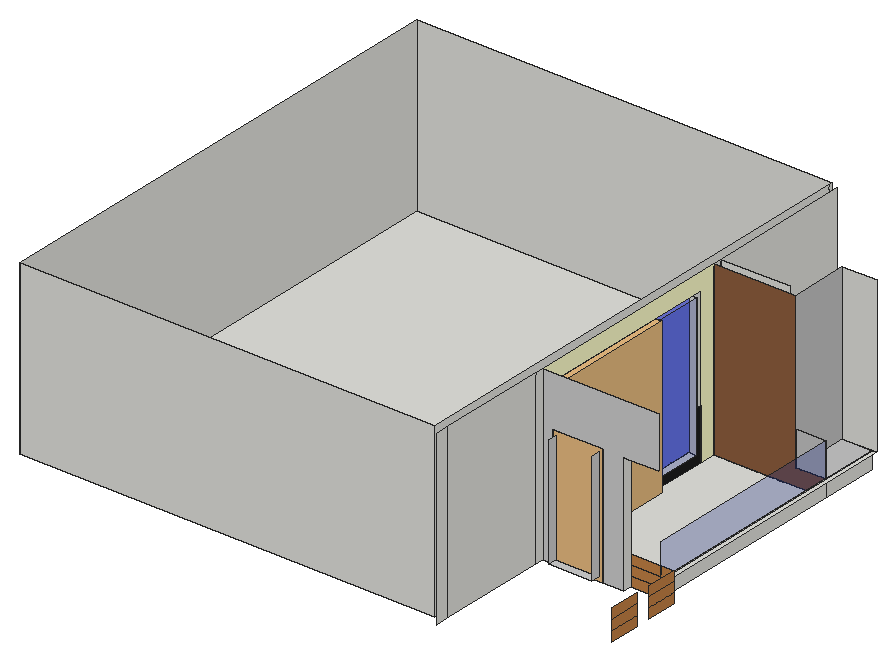
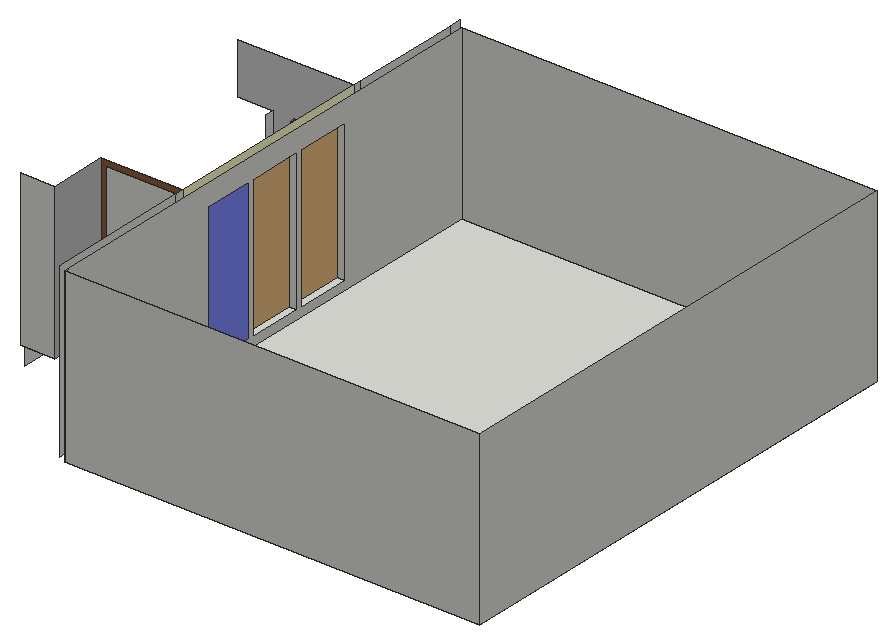
# SketchUp Ruby script. Lengths in inches.
U = 1.inch
M = Sketchup.active_model
def pt(a) = Geom::Point3d.new(a.map { |v| v * U })
def face(e, loops, mat)
  f = e.add_face(loops[0].map { |a| pt(a) })
  loops[1..].each { |l| e.add_face(l.map { |a| pt(a) }).erase! }
  f.material = f.back_material = mat if mat
  f
end
# faces: each face lists its corners as indices into pts; further lists are holes
def faces(e, pts, list, mat = nil) = list.each { |f| face(e, (f[0].is_a?(Array) ? f : [f]).map { |l| l.map { |i| pts[i] } }, mat) }
# xy, xz, yz: faces in a plane at the given z, y or x. An outline is a flat list of corners, or four numbers for a rectangle; further outlines are holes
def ring(l) = l.size == 4 ? [[l[0], l[1]], [l[2], l[1]], [l[2], l[3]], [l[0], l[3]]] : l.each_slice(2).to_a
def flat(e, list, mat, &to3) = list.each { |f| face(e, (f[0].is_a?(Array) ? f : [f]).map { |l| ring(l).map { |u, v| to3.(u, v) } }, mat) }
def xy(e, z, list, mat = nil) = flat(e, list, mat) { |x, y| [x, y, z] }
def xz(e, y, list, mat = nil) = flat(e, list, mat) { |x, z| [x, y, z] }
def yz(e, x, list, mat = nil) = flat(e, list, mat) { |y, z| [x, y, z] }
def lines(e, pts, list) = list.each { |a, b| e.add_line(pt(pts[a]), pt(pts[b])) }
# prism: a flat outline (further loops are holes) pulled along v
def prism(e, loops, v, mat = nil)
  f = face(e, loops, mat); d = Geom::Vector3d.new(v.map { |x| x * U })
  f.pushpull(f.normal.samedirection?(d) ? d.length : -d.length)
end
def box(e, o, s, mat = nil) = prism(e, [[o, [o[0] + s[0], o[1], o[2]], [o[0] + s[0], o[1] + s[1], o[2]], [o[0], o[1] + s[1], o[2]]]], [0, 0, s[2]], mat)
def at(x, y, z, deg = 0) = Geom::Transformation.translation(pt([x, y, z])) * Geom::Transformation.rotation(ORIGIN, Z_AXIS, deg.degrees)
def axes(o, x, y, z) = Geom::Transformation.new([*x, 0, *y, 0, *z, 0, *pt(o).to_a, 1])
def part(name) = M.definitions.add(name)
# library, detail: a bought-in or finely detailed component or shape, given as its bounding box
def library(name, o, s) = part(name).tap { |d| box(d.entities, o, s) }
def detail(e, o, s) = box(e.add_group.entities, o, s)
def put(e, d, t, mat = nil) = e.add_instance(d, t).tap { |i| i.material = mat if mat }
def group(e, t, mat = nil) = e.add_group.tap { |g| g.transformation = t; g.material = mat if mat }.entities
root = M.entities
M.materials.add("E01_Mint_Frost").color = [255, 255, 204]
M.materials.add("Embossed_Stainless_Steel_2_1K").color = [196, 196, 196]
M.materials.add("Glass_Basic_01").color = [23, 48, 186]
M.materials["Glass_Basic_01"].alpha = 0.25
M.materials.add("I03_Bluebell_Mist").color = [130, 140, 255]
M.materials.add("LightPink_Translucent").color = [144, 107, 117]
M.materials["LightPink_Translucent"].alpha = 0.75
M.materials.add("M08_Obsidian_Black").color = [30, 30, 30]
M.materials.add("Wood_Floor_01_1K").color = [196, 130, 70]
M.materials.add("Wood_Veneer_15_1K").color = [142, 95, 62]
M.materials.add("[Cladding_Siding_White]1").color = [207, 207, 207]
c1 = library("porta+4",[0.2,-5.42,1.33],[46.55,4.72,83.21])
c2 = library("mesh-166",[-1553.69,-2604.3125,-42.18],[1702.88,1401.6,88.28])
c3 = part("blade")
p = [[2.15,0.21,22],[0,0.17,0],[0.09,0.45,0],[2.18,0.31,22],[2.29,0.31,22],[0.38,0.45,0],
  [2.48,0.24,33],[2.49,0.24,33],[2.48,0.22,33]]
faces(c3.entities,p,[[0,1,2,3],[4,5,2,3],[6,3,4,7],[8,0,3,6]])
c4 = part("seeds")
p = [[0.3,-0.1,1.38],[-0.01,-0.03,1.59],[-0.01,-0.03,0.03],[0.14,-0.07,-0.07],[0.29,-0.03,3],[0.15,0.01,3.11]]
faces(c4.entities,p,[[0,1,2,3],[1,0,4,5]],"LightPink_Translucent")
c5 = part("blade with seeds")
put(c5.entities,c3,at(0,0,0))
put(c5.entities,c4,axes([2.4,0.25,30.99],[1.5799,-0.05474,1.17369],[-0.12525,1.92788,0.29478],[-0.07173,-0.02425,1.56792]))
xy(root,276,[[6,6,297,354],[303,93,360,93,360,99,381,99,381,243,303,243],[303,243,351,249]])
xy(root,279,[[312,87,342,93]],"[Cladding_Siding_White]1")
xy(root,282,[[297,108,303,147],[297,150,303,189],[297,192,303,228]])
xy(root,288,[[381,99,384,283.95]])
xy(root,288,[[360,243,381,283.95]],"Embossed_Stainless_Steel_2_1K")
xz(root,6,[[6,276,297,396]])
xz(root,93,[[303,276,303,396,384,396,384,360,360,360,360,276,345,276,345,360,309,360,309,276],[[309,276,345,360],[312,279,342,357]]],"[Cladding_Siding_White]1")
xz(root,99,[[381,276,384,283],[381,283,384,288]])
xz(root,99,[[360,276,381,283],[384,276,390,283],[360,283,381,290],[384,283,384,288,381,288,381,290,390,290,390,283],[360,290,381,297],
  [381,290,390,297]],"Wood_Floor_01_1K")
xz(root,108,[[297,282,303,381]])
xz(root,147,[[297,282,303,381]])
xz(root,150,[[297,282,303,381]])
xz(root,189,[[297,282,303,381]])
xz(root,192,[[297,282,303,381]])
xz(root,228,[[297,282,303,381]])
xz(root,243,[[360,288,381,312]],"Embossed_Stainless_Steel_2_1K")
xz(root,243,[[303,276,381,276,381,288,360,288,360,396,303,396]],"Wood_Veneer_15_1K")
xz(root,249,[[303,276,351,396]])
xz(root,283.95,[[360,288,384,396]])
xz(root,354,[[6,276,297,396]])
yz(root,6,[[6,276,354,396]])
yz(root,297,[[[6,276,351,396],[108,282,147,381],[150,282,189,381],[192,282,228,381]],[351,276,354,396]])
yz(root,297,[[192,282,228,381]],"I03_Bluebell_Mist")
yz(root,303,[[0,276,9,396],[9,276,87,396],[87,276,93,396],[243,276,249,396],[249,276,351,396]])
yz(root,303,[[93,276,192,276,192,312,189,312,189,282,150,282,150,312,147,312,147,282,108,282,108,312,105,312,105,384,231,384,231,276,243,276,243,396,93,396]],"E01_Mint_Frost")
yz(root,303,[[192,282,228,381]],"Glass_Basic_01")
yz(root,303,[[192,276,231,276,231,312,228,312,228,282,192,282]],"M08_Obsidian_Black")
yz(root,312,[[87,279,93,357]],"[Cladding_Siding_White]1")
yz(root,342,[[87,279,93,357]],"[Cladding_Siding_White]1")
yz(root,360,[[93,276,99,360]])
yz(root,360,[[243,288,283.95,396]],"Embossed_Stainless_Steel_2_1K")
yz(root,381,[[99,276,243,288],[243,276,283.95,288]])
yz(root,381,[[99,288,243,312]],"Glass_Basic_01")
yz(root,390,[[45,276,66.6,283],[77.4,276,99,283],[45,283,66.6,290],[77.4,283,99,290],[45,290,66.6,297],
  [77.4,290,99,297]],"Wood_Floor_01_1K")
p = [[303,231,312],[303,231,276]]
lines(root,p,[[0,1]])
put(root,c1,axes([310,97.01,274.61],[0.74,0,0],[0,0.74,0],[0,0,1.01007]))
g1 = group(root,at(305.35,127.3,410.45))
put(g1,c2,axes([-0.18,-15.08,66.23],[0,-0.05118,0],[0,0,0.07706],[-0.05118,0,0]))
put(root,c5,axes([329.04,108.57,288.76],[-0.2011,-0.61905,-0.65645],[0.5793,-0.22295,-0.17229],[-0.02223,-0.20963,1.449]))
put(root,c5,axes([330.88,109.625,288.76],[0.17956,0.55272,-0.65059],[-0.51723,0.19906,-0.17075],[0.01985,0.18717,1.43607]))
put(root,c5,axes([330.82,108.47,288.73],[0.50939,0.09897,-0.58612],[-0.10749,0.61051,-0.15383],[0.15202,0.07398,1.29375]))
put(root,c5,axes([329.12,109.73,288.73],[-0.50939,-0.09897,-0.58612],[0.10749,-0.61051,-0.15383],[-0.15202,-0.07398,1.29375]))
put(root,c5,axes([329.92,107.9375,288.73],[0.32983,-0.45375,-0.58612],[0.40974,0.41145,-0.15383],[0.13217,-0.11319,1.29375]))
put(root,c5,axes([330.02,110.26,288.73],[-0.32983,0.45375,-0.58612],[-0.40974,-0.41145,-0.15383],[-0.13217,0.11319,1.29375]))
put(root,c5,axes([331.49,107.3125,288.6875],[0.4583,0.30184,-0.46672],[-0.27394,0.54125,0],[0.10438,0.06875,1.48054]))
put(root,c5,axes([330.57,111.5,288.6875],[-0.4583,0.30184,-0.46672],[-0.27394,-0.54125,0],[-0.10438,0.06875,1.48054]))
put(root,c5,axes([327.85,108.49,288.6875],[0,-0.60368,-0.46672],[0.54787,0,0],[0,-0.13749,1.48054]))
put(root,c5,axes([328.45,110.89,288.6875],[-0.4583,-0.30184,-0.46672],[0.27394,-0.54125,0],[-0.10438,-0.06875,1.48054]))
put(root,c5,axes([329.375,106.7,288.6875],[0.4583,-0.30184,-0.46672],[0.27394,0.54125,0],[0.10438,-0.06875,1.48054]))
put(root,c5,axes([332.09,109.71,288.6875],[0,0.60368,-0.46672],[-0.54787,0,0],[0,0.13749,1.48054]))
put(root,c5,axes([329.34,108.73,288.87],[0.23759,-0.54397,-0.42055],[0.49367,0.26179,0.2024],[0,-0.12539,1.35025]))
put(root,c5,axes([329.38,109.54,288.87],[-0.29417,-0.5067,-0.42055],[0.44558,-0.35681,0.2024],[-0.0952,-0.0627,1.35025]))
put(root,c5,axes([330.5625,108.66,288.87],[0.29417,0.5067,-0.42055],[-0.44558,0.35681,0.2024],[0.0952,0.0627,1.35025]))
put(root,c5,axes([330.6,109.46,288.87],[-0.23759,0.54397,-0.42055],[-0.49367,-0.26179,0.2024],[0,0.12539,1.35025]))
put(root,c5,axes([330.01,109.9,288.87],[-0.53176,0.03727,-0.42055],[-0.04809,-0.6186,0.2024],[-0.0952,0.0627,1.35025]))
put(root,c5,axes([329.48,106.9375,288.7],[0.45686,0.14937,-0.29119],[-0.11503,0.52602,0.29119],[0.0921,-0.06066,1.30635]))
put(root,c5,axes([331.85,109.69,288.7],[-0.34183,0.37665,-0.29119],[-0.34183,-0.37665,0.29119],[0,0.12132,1.30635]))
put(root,c5,axes([328.58,110.66,288.7],[-0.11503,-0.52602,-0.29119],[0.45686,-0.14937,0.29119],[-0.0921,-0.06066,1.30635]))
put(root,c5,axes([330.46,111.26,288.7],[-0.45686,-0.14937,-0.29119],[0.11503,-0.52602,0.29119],[-0.0921,0.06066,1.30635]))
put(root,c5,axes([331.37,107.54,288.7],[0.11503,0.52602,-0.29119],[-0.45686,0.14937,0.29119],[0.0921,0.06066,1.30635]))
put(root,c5,axes([328.09,108.5,288.7],[0.34183,-0.37665,-0.29119],[0.34183,0.37665,0.29119],[0,-0.12132,1.30635]))
put(root,c5,axes([331.47,111.61,288.2],[0.03568,-0.08715,1.65762],[0.44916,-0.25668,-0.25323],[0.13617,0.13285,0.28235]))
put(root,c5,axes([327.48,108.87,288.2],[0.01242,0.09514,1.65762],[-0.25036,0.49684,-0.25323],[-0.17783,-0.02504,0.28235]))
put(root,c5,axes([329.72,105.64,288.2],[-0.08214,0.02175,1.65762],[-0.45422,-0.24483,-0.25323],[0.00762,-0.20421,0.28235]))
put(root,c5,axes([329.37,111.59,288.2],[0.07925,-0.03285,1.65762],[0.47671,0.18081,-0.25323],[0.01394,0.20378,0.28235]))
put(root,c5,axes([332.76,108.96,288.2],[-0.02559,-0.09165,1.65762],[0.1775,-0.53611,-0.25323],[0.17905,-0.00771,0.28235]))
put(root,c5,axes([328.25,106.39,288.2],[-0.04743,0.07953,1.65762],[-0.47936,0.17146,-0.25323],[-0.1158,-0.15598,0.28235]))
put(root,c5,axes([327.35,111.53,288.2],[0.06569,0.06031,1.65762],[0.11138,0.55882,-0.25323],[-0.14558,0.11917,0.28235]))
put(root,c5,axes([331.73,106.68,288.2],[-0.07329,-0.04756,1.65762],[-0.18827,-0.53132,-0.25323],[0.127,-0.14418,0.28235]))
put(root,c5,axes([329,108.02,288.29],[-0.482,0.24169,1.21193],[-0.15342,-0.69348,0.47091],[0.29598,0.01154,1.37843]))
put(root,c5,axes([330.38,109.73,289.3],[0.05706,0.68884,-0.2735],[-0.59432,0.04165,-0.47002],[-0.10465,0.09176,1.50125]))
put(root,c5,axes([330.66,109.01,289.3],[0.55148,0.28805,-0.2735],[-0.26554,0.60796,-0.47002],[0.01733,0.14927,1.50125]))
put(root,c5,axes([329.29,109.1875,289.3],[-0.55148,-0.28805,-0.2735],[0.26554,-0.60796,-0.47002],[-0.01733,-0.14927,1.50125]))
put(root,c5,axes([329.5625,108.46,289.3],[-0.05706,-0.68884,-0.2735],[0.59432,-0.04165,-0.47002],[0.10465,-0.09176,1.50125]))
put(root,c5,axes([330.25,108.375,289.3],[0.49442,-0.40079,-0.2735],[0.32878,0.56631,-0.47002],[0.12199,0.05751,1.50125]))
put(root,c5,axes([329.69,109.82,289.3],[-0.49442,0.40079,-0.2735],[-0.32878,-0.56631,-0.47002],[-0.12199,-0.05751,1.50125]))
put(root,c5,axes([330.55,110.42,288.85],[0.51411,-0.20483,-0.18046],[0.18065,0.59003,0.00007],[0.05675,-0.02264,1.63463]))
put(root,c5,axes([330.25,110,289.11],[-0.47817,-0.48589,-0.23681],[0.40236,-0.54561,0.51822],[-0.12876,0.05684,1.58123]))
put(root,c5,axes([329.42,109.83,289.08],[0.12979,-0.71533,-0.22023],[0.6154,0.12469,0.48194],[-0.10753,-0.09879,1.47054]))
put(root,c5,axes([329.63,106.07,288.79],[-0.3384,0.34633,-0.03659],[-0.31006,-0.3793,-0.1659],[-0.02183,-0.10747,0.54722]))
put(root,c5,axes([327.95,106.7,288.79],[-0.14126,0.49294,-0.03659],[-0.43477,-0.15163,-0.1659],[-0.06601,-0.08063,0.54722]))
put(root,c5,axes([332.99,108.83,288.92],[-0.3036,-0.38602,-0.06098],[0.3325,-0.3537,-0.27651],[0.09421,-0.0249,0.91203]))
put(root,c5,axes([332.42,109.34,288.65],[-0.3154,0.07245,1.33088],[-0.0502,-0.57666,0.07618],[0.2209,-0.08728,0.75732]))
put(root,c5,axes([330.6,111.33,288.85],[-0.30235,-0.60704,-0.04834],[0.51222,-0.33735,0.48511],[-0.12622,0.0578,1.53813]))
put(root,c5,axes([331.98,109.6,288.86],[-0.61202,-0.00483,-0.04678],[0,-0.67471,0.46946],[-0.01923,0.15359,1.48851]))
put(root,c5,axes([330.22,110.51,288.95],[0.2129,0.69353,-0.05652],[-0.60833,0.24302,0],[0.00743,0.02422,1.61843]))
put(root,c5,axes([330.36,109.42,288.95],[-0.45549,-0.5196,-0.05763],[0.45577,-0.51991,0],[-0.01591,-0.01814,1.65037]))
put(root,c5,axes([330.52,109.16,288.95],[0,0.69816,-0.05299],[-0.61233,0,0],[0,0.02194,1.68606]))
put(root,c5,axes([328.96,106.79,289.02],[-0.30616,-0.60492,0],[0.51222,-0.33735,-0.48511],[0.11666,-0.07683,1.53889]))
put(root,c5,axes([328.73,111.25,289.02],[-0.30616,0.60492,0],[-0.51222,-0.33735,-0.48511],[-0.11666,-0.07683,1.53889]))
put(root,c5,axes([330.98,111.4,289.02],[0.30616,0.60492,0],[-0.51222,0.33735,-0.48511],[-0.11666,0.07683,1.53889]))
put(root,c5,axes([327.72,108.95,289.02],[-0.61233,0,0],[0,-0.67471,-0.48511],[0,-0.15367,1.53889]))
put(root,c5,axes([331.21,106.95,289.03],[0.30616,-0.60492,0],[0.51222,0.33735,-0.48511],[0.11666,0.07683,1.53889]))
put(root,c5,axes([332.23,109.25,289.03],[0.61233,0,0],[0,0.67471,-0.48511],[0,0.15367,1.53889]))
put(root,c5,axes([328.19,108.77,288.98],[-0.45549,0.50754,0.28911],[-0.45577,-0.5022,-0.34302],[-0.01591,-0.14413,1.54992]))
put(root,c5,axes([330.61,111.02,288.98],[0.61306,0.19622,0.28911],[-0.15337,0.70136,-0.34302],[-0.10147,0.08778,1.54992]))
put(root,c5,axes([329.84,110.72,288.86],[-0.49367,-0.27103,0],[0.23759,-0.56315,0],[0,0,1.52945]))
put(root,c5,axes([330.4,110.73,288.86],[0.49367,0.27103,0],[-0.23759,0.56315,0],[0,0,1.64456]))
put(root,c5,axes([329.95,110.49,288.86],[-0.15978,-0.52046,0],[0.45625,-0.18226,0],[0,0,1.45109]))
put(root,c5,axes([330.21,108.875,288.86],[0,-0.69851,0],[0.61233,0,0],[0,0,1.68689]))
put(root,c5,axes([330.625,109.03,288.87],[0.54787,0,0],[0,0.62498,0],[0,0,1.67702]))
put(root,c5,axes([330.61,109.3,288.875],[0.34183,0.38994,0],[-0.34183,0.38994,0],[0,0,1.5911]))
put(root,c5,axes([329.5,109.48,289.01],[0.61893,0.12719,0.43009],[-0.12596,0.71835,0.16877],[-0.09045,-0.06936,1.49325]))
put(root,c5,axes([329.92,108.4375,289.01],[-0.40602,0.54785,0.43009],[-0.48237,-0.48361,0.16877],[0.09788,-0.05467,1.49325]))
put(root,c5,axes([329.44,108.82,289.01],[0.2129,0.67504,0.43009],[-0.60833,0.23474,0.16877],[0.00743,-0.12404,1.49325]))
put(root,c5,axes([330.45,108.71,289.03],[-0.61893,-0.12719,0.46247],[0.12596,-0.71835,0.18148],[0.09045,0.06936,1.60565]))
put(root,c5,axes([329.64,109,289.08],[0.55175,0.29259,0.22621],[-0.26554,0.60796,0.47002],[0,-0.14015,1.5091]))
put(root,c5,axes([330.49,109.87,289.25],[0.36178,0.36271,0.13611],[-0.30177,0.40921,-0.38866],[-0.084,0.05532,1.1914]))
put(root,c5,axes([330.29,108.2,289.25],[0.09447,-0.53876,0.13611],[0.46155,0.09352,-0.38866],[0.084,0.05532,1.1914]))
put(root,c5,axes([330.8125,108.97,289.25],[0.45625,-0.17605,0.13611],[0.15978,0.50273,-0.38866],[0,0.11064,1.1914]))
put(root,c5,axes([329.65,109.99,289.25],[-0.09447,0.53876,0.13611],[-0.46155,-0.09352,-0.38866],[-0.084,-0.05532,1.1914]))
put(root,c5,axes([328.28,111.67,289.45],[0.44486,-0.1069,0.06117],[0.10227,0.43069,-0.81126],[-0.0282,0.21802,0.72719]))
put(root,c5,axes([327.82,107.74,289.23],[0.09561,0.16807,1.34422],[-0.22031,0.45686,-0.28909],[-0.22622,-0.1092,0.57472]))
put(root,c5,axes([328.17,112.125,289.23],[0.15453,-0.09523,1.34422],[0.38153,0.28715,-0.28909],[-0.11356,0.24846,0.57472]))
put(root,c5,axes([330.41,110.78,289.23],[0.00864,-0.20012,1.34422],[0.41296,-0.22353,-0.28909],[0.12748,0.23952,0.57472]))
put(root,c5,axes([330.75,106.31,289.23],[-0.13919,0.12219,1.34422],[-0.41687,-0.21387,-0.28909],[0.07727,-0.26598,0.57472]))
put(root,c5,axes([332.1,107.74,289.23],[-0.17494,-0.01788,1.34422],[-0.17922,-0.47967,-0.28909],[0.21491,-0.13569,0.57472]))
put(root,c5,axes([328.6,106.07,289.23],[-0.02965,0.19748,1.34422],[-0.43351,0.16532,-0.28909],[-0.10133,-0.25525,0.57472]))
put(root,c5,axes([332.51,110.19,289.23],[-0.11793,-0.14847,1.34422],[0.15345,-0.49116,-0.28909],[0.23861,0.06653,0.57472]))
put(root,c5,axes([327.16,110.19,289.23],[0.17018,0.04956,1.34422],[0.10969,0.50618,-0.28909],[-0.23117,0.09475,0.57472]))
put(root,c5,axes([330.78,107.57,289.12],[-0.52621,0.16023,0.16584],[-0.12993,-0.59629,0.32981],[0.04693,0.08688,1.50782]))
put(root,c5,axes([331.54,109.13,289.12],[-0.38474,-0.43973,0.16584],[0.38772,-0.42651,0.32981],[-0.04249,0.0898,1.50782]))
put(root,c5,axes([329.21,107.53,289.12],[-0.14146,0.59996,0.16584],[-0.51766,-0.16978,0.32981],[0.08942,-0.00292,1.50782]))
put(root,c5,axes([330.73,110.66,289.12],[0.14146,-0.59996,0.16584],[0.51766,0.16978,0.32981],[-0.08942,0.00292,1.50782]))
put(root,c5,axes([329.16,110.63,289.12],[0.52621,-0.16023,0.16584],[0.12993,0.59629,0.32981],[-0.04693,-0.08688,1.50782]))
put(root,c5,axes([328.09,109.05,289.12],[0,0.60368,0.46672],[-0.54787,0,0],[0,-0.13749,1.48054]))
put(root,c5,axes([330.95,107.26,289.12],[-0.4583,-0.30184,0.46672],[0.27394,-0.54125,0],[0.10438,0.06875,1.48054]))
put(root,c5,axes([331.85,109.15,289.12],[0,-0.60368,0.46672],[0.54787,0,0],[0,0.13749,1.48054]))
put(root,c5,axes([330.875,110.98,289.12],[0.4583,-0.30184,0.46672],[0.27394,0.54125,0],[-0.10438,0.06875,1.48054]))
put(root,c5,axes([328.99,110.93,289.12],[0.4583,0.30184,0.46672],[-0.27394,0.54125,0],[-0.10438,-0.06875,1.48054]))
put(root,c5,axes([330.61,108.84,289.35],[0.23759,-0.54397,0.42055],[0.49367,0.26179,-0.2024],[0,0.12539,1.35025]))
put(root,c5,axes([329.46,108.6,289.35],[-0.53176,0.03727,0.42055],[-0.04809,-0.6186,-0.2024],[0.0952,-0.0627,1.35025]))
put(root,c5,axes([330.1,108.34,289.35],[-0.29417,-0.5067,0.42055],[0.44558,-0.35681,-0.2024],[0.0952,0.0627,1.35025]))
put(root,c5,axes([329.34,109.35,289.35],[-0.23759,0.54397,0.42055],[-0.49367,-0.26179,-0.2024],[0,-0.12539,1.35025]))
put(root,c5,axes([330.48,109.6,289.35],[0.53176,-0.03727,0.42055],[0.04809,0.6186,-0.2024],[-0.0952,0.0627,1.35025]))
put(root,c5,axes([331.4375,111.75,289.3],[-0.31402,-0.01893,0.98757],[0.20738,-0.40212,0.54525],[0.12405,0.14286,0.77466]))
put(root,c5,axes([327.25,108.24,289.39],[0.31263,-0.0432,1.07969],[-0.19831,0.38061,0.79328],[-0.15449,-0.0571,0.23781]))
put(root,c5,axes([331.39,110.96,289.39],[-0.27572,-0.17358,1.07969],[0.35602,-0.17637,0.79328],[0.09603,0.1494,0.23781]))
put(root,c5,axes([326.81,111.25,289.39],[0.20408,-0.2736,1.07969],[0.08053,0.43313,0.79328],[-0.14748,0.07756,0.23781]))
put(root,c5,axes([333.08,109.53,289.39],[-0.30256,0.09966,1.07969],[0.14242,-0.41189,0.79328],[0.16051,0.02818,0.23781]))
put(root,c5,axes([328.45,105.76,289.39],[0.25544,0.21011,1.07969],[-0.37201,0.1263,0.79328],[-0.0796,-0.16148,0.23781]))
put(root,c5,axes([328.54,112.44,289.39],[-0.01267,-0.35895,1.07969],[0.31667,0.25602,0.79328],[-0.06228,0.17109,0.23781]))
put(root,c5,axes([332.3,106.86,289.39],[-0.16311,0.3073,1.07969],[-0.1402,-0.41288,0.79328],[0.13471,-0.10346,0.23781]))
put(root,c5,axes([330.24,105.33,289.39],[0.06282,0.35202,1.07969],[-0.34848,-0.19497,0.79328],[0.0375,-0.18025,0.23781]))
put(root,c5,axes([330.72,109.01,289.46],[-0.01338,-0.56839,1.32796],[0.60542,0.14734,0.56227],[-0.14319,0.31102,1.25349]))
put(root,c5,axes([329.07,106.87,291.47],[-0.41756,-0.29179,-0.66783],[0.29675,-0.51132,0.08059],[-0.15128,-0.17422,0.9447]))
put(root,c5,axes([329.52,111.35,291.47],[0.23372,0.49086,-0.66783],[-0.48111,0.27356,0.08059],[0.05465,0.23717,0.9447]))
put(root,c5,axes([328.22,107.59,291.47],[-0.48951,-0.01454,-0.66783],[0.03288,-0.61207,0.08059],[-0.20738,-0.06459,0.9447]))
put(root,c5,axes([331.72,108.18,291.47],[0.25579,-0.47633,-0.66783],[0.44823,0.33852,0.08059],[0.15273,-0.17258,0.9447]))
put(root,c5,axes([331.85,109.38,291.47],[0.4303,-0.26662,-0.66783],[0.23981,0.54882,0.08059],[0.20791,-0.06234,0.9447]))
put(root,c5,axes([331.09,107.21,291.47],[0.01274,-0.55841,-0.66783],[0.53656,0.0375,0.08059],[0.05662,-0.23657,0.9447]))
put(root,c5,axes([331.43,110.49,291.47],[0.48951,0.01454,-0.66783],[-0.03288,0.61207,0.08059],[0.20738,0.06459,0.9447]))
put(root,c5,axes([330.12,106.73,291.47],[-0.23372,-0.49086,-0.66783],[0.48111,-0.27356,0.08059],[-0.05465,-0.23717,0.9447]))
put(root,c5,axes([329.7,111.45,291.19],[0.48137,0.15133,-0.48033],[-0.165,0.51886,-0.37205],[0.04414,0.2089,0.91906]))
put(root,c5,axes([330.98,107.02,291.19],[-0.35055,-0.40562,-0.48033],[0.37031,-0.35523,-0.37205],[0.05334,-0.20609,0.91906]))
put(root,c5,axes([328.87,106.88,291.19],[-0.48321,0.1435,-0.48033],[-0.08453,-0.54345,-0.37205],[-0.12979,-0.15574,0.91906]))
put(root,c5,axes([331.93,109.18,291.19],[0.13266,-0.54912,-0.48033],[0.45484,0.18822,-0.37205],[0.18313,-0.05035,0.91906]))
put(root,c5,axes([328.05,107.71,291.19],[-0.35558,0.39989,-0.48033],[-0.31141,-0.42243,-0.37205],[-0.18066,-0.06084,0.91906]))
put(root,c5,axes([327.93,110.125,291.19],[0.1258,0.55122,-0.48033],[-0.4764,0.09643,-0.37205],[-0.13652,0.14806,0.91906]))
put(root,c5,axes([327.71,108.9,291.19],[-0.13266,0.54912,-0.48033],[-0.45484,-0.18822,-0.37205],[-0.18313,0.05035,0.91906]))
put(root,c5,axes([329.94,106.63,291.19],[-0.48137,-0.15133,-0.48033],[0.165,-0.51886,-0.37205],[-0.04414,-0.2089,0.91906]))
put(root,c5,axes([331.71,107.96,291.19],[-0.1258,-0.55122,-0.48033],[0.4764,-0.09643,-0.37205],[0.13652,-0.14806,0.91906]))
put(root,c5,axes([330.77,111.2,291.19],[0.48321,-0.1435,-0.48033],[0.08453,0.54345,-0.37205],[0.12979,0.15574,0.91906]))
put(root,c5,axes([328.55,110.875,291.81],[-0.01274,0.55841,-0.74129],[-0.53656,-0.0375,0.08946],[-0.05662,0.23657,1.04862]))
put(root,c5,axes([328.66,111.06,291.5],[0.35055,0.40562,-0.53317],[-0.37031,0.35523,-0.41298],[-0.05334,0.20609,1.02016]))
put(root,c5,axes([330.07,110.17,289.92],[0.42317,0.24343,1.42185],[-0.41456,0.52443,0.56227],[-0.18569,-0.31082,1.19198]))
put(root,c5,axes([328.67,108.57,289.93],[0.13919,-0.08733,1.6644],[0.048,0.60974,0.13026],[-0.3015,0.08091,0.59487]))
put(root,c5,axes([328.37,111.66,289.95],[0.01076,-0.31164,1.45085],[0.48391,0.16461,0.20049],[-0.04193,0.33214,0.68509]))
put(root,c5,axes([331.72,110.74,291.05],[0.27863,0.37797,-0.33289],[-0.31815,0.35779,0.42977],[0.16164,0.05444,0.82232]))
put(root,c5,axes([327.43,108.65,291.05],[-0.40696,-0.16841,-0.33289],[0.1187,-0.49132,0.42977],[-0.16385,0.04505,0.82232]))
put(root,c5,axes([327.58,110.07,291.05],[-0.42626,0.08628,-0.33289],[-0.11256,-0.4932,0.42977],[-0.12215,0.13247,0.82232]))
put(root,c5,axes([332.21,109.43,291.05],[0.40696,0.16841,-0.33289],[-0.1187,0.49132,0.42977],[0.16385,-0.04505,0.82232]))
put(root,c5,axes([328.92,106.48,291.05],[-0.07563,-0.48625,-0.33289],[0.43235,-0.1284,0.42977],[-0.11613,-0.13934,0.82232]))
put(root,c5,axes([328.33,111.21,291.05],[-0.33133,0.31784,-0.33289],[-0.31365,-0.36292,0.42977],[-0.04772,0.1844,0.82232]))
put(root,c5,axes([332.0625,108.02,291.05],[0.42626,-0.08628,-0.33289],[0.11256,0.4932,0.42977],[0.12215,-0.13247,0.82232]))
put(root,c5,axes([329.48,111.77,291.05],[-0.14763,0.46424,-0.33289],[-0.4307,-0.1354,0.42977],[0.03949,0.18691,0.82232]))
put(root,c5,axes([331.3125,106.875,291.05],[0.33133,-0.31784,-0.33289],[0.31365,0.36292,0.42977],[0.04772,-0.1844,0.82232]))
put(root,c5,axes([330.16,106.3125,291.05],[0.14763,-0.46424,-0.33289],[0.4307,0.1354,0.42977],[-0.03949,-0.18691,0.82232]))
put(root,c5,axes([327.92,107.34,291.05],[-0.27863,-0.37797,-0.33289],[0.31815,-0.35779,0.42977],[-0.16164,-0.05444,0.82232]))
put(root,c5,axes([332.55,110.8,290.49],[-0.09372,-0.50747,-0.03282],[0.44299,-0.11666,-0.14882],[0.09251,0.03217,0.49085]))
put(root,c5,axes([330.72,109.78,290.44],[-0.1819,-0.10401,1.61094],[0.37643,-0.43634,0.13026],[0.23461,0.19684,0.68866]))
put(root,c5,axes([330.49,106.93,290.44],[-0.09118,0.2075,1.61094],[-0.3825,-0.42941,0.13026],[0.17255,-0.26763,0.68866]))
put(root,c5,axes([331.1,108.82,290.44],[-0.20312,0.01367,1.61094],[0.13474,-0.59258,0.13026],[0.28946,0.03665,0.68866]))
put(root,c5,axes([329.97,110.38,290.44],[-0.11194,-0.19382,1.61094],[0.51725,-0.16318,0.13026],[0.1169,0.30428,0.68866]))
put(root,c5,axes([329.06,110.48,290.44],[-0.01199,-0.2317,1.61094],[0.51947,0.15371,0.13026],[-0.03213,0.3302,0.68866]))
put(root,c5,axes([328.22,110.04,290.44],[0.09118,-0.2075,1.61094],[0.3825,0.42941,0.13026],[-0.17255,0.26763,0.68866]))
put(root,c5,axes([327.69,109.18,290.44],[0.16991,-0.12769,1.61094],[0.14304,0.59005,0.13026],[-0.26674,0.13336,0.68866]))
put(root,c5,axes([328.3125,109.58,290.44],[0.12231,-0.18549,1.61094],[0.30882,0.50067,0.13026],[-0.21182,0.22801,0.68866]))
put(root,c5,axes([328.74,106.59,290.44],[0.11194,0.19382,1.61094],[-0.51725,0.16318,0.13026],[-0.1169,-0.30428,0.68866]))
put(root,c5,axes([327.99,107.19,290.44],[0.1819,0.10401,1.61094],[-0.37643,0.43634,0.13026],[-0.23461,-0.19684,0.68866]))
put(root,c5,axes([327.61,108.14,290.44],[0.20312,-0.01367,1.61094],[-0.13474,0.59258,0.13026],[-0.28946,-0.03665,0.68866]))
put(root,c5,axes([331.4,110.79,291.52],[0.02622,-0.61393,-0.11431],[0.49645,0.01678,-0.63445],[0.1912,0.04265,0.96403]))
put(root,c5,axes([327.6875,108.43,291.52],[0.24639,0.54664,-0.11431],[-0.43729,0.26863,-0.63445],[-0.18428,0.07212,0.96403]))
put(root,c5,axes([331.35,107.24,291.52],[-0.53819,-0.02991,-0.11431],[0.01471,-0.56632,-0.63445],[0.03738,-0.21811,0.96403]))
put(root,c5,axes([331.96,109.65,291.52],[-0.24639,-0.54664,-0.11431],[0.43729,-0.26863,-0.63445],[0.18428,-0.07212,0.96403]))
put(root,c5,axes([329.29,111.48,291.52],[0.47919,-0.28106,-0.11431],[0.23549,0.49884,-0.63445],[0.06322,0.21021,0.96403]))
put(root,c5,axes([328.24,107.3,291.52],[-0.02622,0.61393,-0.11431],[-0.49645,-0.01678,-0.63445],[-0.1912,-0.04265,0.96403]))
put(root,c5,axes([330.42,111.46,291.52],[0.2918,-0.51673,-0.11431],[0.42258,0.29769,-0.63445],[0.14689,0.14599,0.96403]))
put(root,c5,axes([327.7,109.73,291.52],[0.45297,0.33287,-0.11431],[-0.26096,0.48206,-0.63445],[-0.12798,0.16757,0.96403]))
put(root,c5,axes([330.36,106.61,291.52],[-0.47919,0.28106,-0.11431],[-0.23549,-0.49884,-0.63445],[-0.06322,-0.21021,0.96403]))
put(root,c5,axes([331.9375,108.35,291.52],[-0.45297,-0.33287,-0.11431],[0.26096,-0.48206,-0.63445],[0.12798,-0.16757,0.96403]))
put(root,c5,axes([330.75,108.41,291],[-0.42314,-0.31366,1.29986],[0.4468,-0.48836,0.56085],[0.13652,0.29431,1.25644]))
put(root,c5,axes([327.17,108.98,291.22],[-0.07997,0.07838,1.64448],[0.0068,0.57266,-0.26007],[-0.1833,0.07447,0.13189]))
put(root,c5,axes([333.29,108.8,291.22],[0.06795,-0.09195,1.64448],[-0.08698,-0.56405,-0.26007],[0.1705,-0.10694,0.13189]))
put(root,c5,axes([331.83,110.42,291.22],[0.10505,-0.01021,1.64448],[0.28813,-0.469,-0.26007],[0.18685,0.06191,0.13189]))
put(root,c5,axes([331.84,106.34,291.22],[-0.00473,-0.12015,1.64448],[-0.39924,-0.34724,-0.26007],[0.06173,-0.21049,0.13189]))
put(root,c5,axes([327.19,111.11,291.22],[-0.01217,0.11946,1.64448],[0.34544,0.41559,-0.26007],[-0.09043,0.19653,0.13189]))
put(root,c5,axes([329.17,112.59,291.22],[0.06207,0.09721,1.64448],[0.50093,0.03819,-0.26007],[0.05037,0.21439,0.13189]))
put(root,c5,axes([329.59,105.3,291.22],[-0.0749,-0.08464,1.64448],[-0.49984,0.05366,-0.26007],[-0.07977,-0.20245,0.13189]))
put(root,c5,axes([327.96,106.23,291.22],[-0.10536,-0.00426,1.64448],[-0.33544,0.42612,-0.26007],[-0.17898,-0.08707,0.13189]))
put(root,c5,axes([327.55,106.59,291.22],[0.0363,0.06025,1.6674],[-0.17501,0.54156,-0.15755],[-0.17724,0.00392,0.29507]))
put(root,c5,axes([329.08,105.02,291.22],[-0.00914,0.07236,1.6674],[-0.45057,0.26261,-0.15755],[-0.13259,-0.13424,0.29507]))
put(root,c5,axes([330.04,111.88,291.22],[0.00145,-0.07309,1.6674],[0.41965,-0.32245,-0.15755],[0.14577,0.11509,0.29507]))
put(root,c5,axes([326.28,109.56,291.22],[0.06249,0.01619,1.6674],[0.19333,0.53339,-0.15755],[-0.12793,0.14,0.29507]))
put(root,c5,axes([333.05,108.21,291.22],[-0.06396,-0.00458,1.6674],[-0.2656,-0.49127,-0.15755],[0.10666,-0.16153,0.29507]))
put(root,c5,axes([332.94,111.28,291.22],[-0.04428,-0.05285,1.6674],[0.09686,-0.56651,-0.15755],[0.17442,-0.03619,0.29507]))
put(root,c5,axes([327.15,112.34,291.22],[0.05555,-0.03645,1.6674],[0.45917,0.24243,-0.15755],[-0.01079,0.20185,0.29507]))
put(root,c5,axes([331.73,105.91,291.22],[-0.04973,0.04611,1.6674],[-0.48725,-0.15557,-0.15755],[-0.01764,-0.20123,0.29507]))
put(root,c5,axes([328.29,110.85,291.87],[0.53819,0.02991,-0.12688],[-0.01471,0.56632,-0.70424],[-0.03738,0.21811,1.07008]))
put(root,c5,axes([329.21,106.4,291.9],[-0.32682,0.57873,-0.12802],[-0.47329,-0.33342,-0.71058],[-0.16452,-0.16351,1.07972]))
put(root,c5,axes([329.11,106.4375,291.24],[0.22256,-0.38349,0.06044],[0.31694,0.22327,0.47584],[-0.10247,-0.12295,0.72558]))
put(root,c5,axes([329.3,111.7,291.24],[-0.36083,0.20517,0.06044],[-0.17661,-0.37413,0.47584],[0.03485,0.16492,0.72558]))
put(root,c5,axes([332.1,108.23,291.24],[0.33617,0.25389,0.06044],[-0.19572,0.36154,0.47584],[0.10778,-0.11689,0.72558]))
put(root,c5,axes([332.15,109.64,291.24],[0.17985,0.41162,0.06044],[-0.32797,0.20147,0.47584],[0.14457,-0.03975,0.72558]))
put(root,c5,axes([328.0625,107.19,291.24],[0.02466,-0.45905,0.06044],[0.37234,0.01259,0.47584],[-0.14263,-0.04803,0.72558]))
put(root,c5,axes([331.44,107.04,291.24],[0.40242,0.02813,0.06044],[-0.01103,0.42474,0.47584],[0.04211,-0.1627,0.72558]))
put(root,c5,axes([331.58,110.89,291.24],[-0.02466,0.45905,0.06044],[-0.37234,-0.01259,0.47584],[0.14263,0.04803,0.72558]))
put(root,c5,axes([327.54,109.85,291.24],[-0.33617,-0.25389,0.06044],[0.19572,-0.36154,0.47584],[-0.10778,0.11689,0.72558]))
put(root,c5,axes([330.35,106.38,291.24],[0.36083,-0.20517,0.06044],[0.17661,0.37413,0.47584],[-0.03485,-0.16492,0.72558]))
put(root,c5,axes([327.49,108.44,291.24],[-0.17985,-0.41162,0.06044],[0.32797,-0.20147,0.47584],[-0.14457,0.03975,0.72558]))
put(root,c5,axes([330.53,111.64,291.24],[-0.22256,0.38349,0.06044],[-0.31694,-0.22327,0.47584],[0.10247,0.12295,0.72558]))
put(root,c5,axes([328.2,111.05,291.24],[-0.40242,-0.02813,0.06044],[0.01103,-0.42474,0.47584],[-0.04211,0.1627,0.72558]))
put(root,c5,axes([330.22,106.42,291.24],[0.48252,0.15782,0.45122],[-0.165,0.51886,0.37205],[-0.029,-0.20404,0.9337]))
put(root,c5,axes([331.61,110.74,291.24],[-0.36108,0.39778,0.45122],[-0.31141,-0.42243,0.37205],[0.1694,0.07337,0.9337]))
put(root,c5,axes([332.12,109.49,291.24],[-0.13835,0.55043,0.45122],[-0.45484,-0.18822,0.37205],[0.17887,-0.03308,0.9337]))
put(root,c5,axes([327.63,109.96,291.24],[-0.12145,-0.5556,0.45122],[0.4764,-0.09643,0.37205],[-0.14041,0.13067,0.9337]))
put(root,c5,axes([328.33,111.09,291.24],[-0.3487,-0.41189,0.45122],[0.37031,-0.35523,0.37205],[-0.06432,0.19325,0.9337]))
put(root,c5,axes([331.3125,107,291.24],[0.3487,0.41189,0.45122],[-0.37031,0.35523,0.37205],[0.06432,-0.19325,0.9337]))
put(root,c5,axes([327.52,108.59,291.24],[0.13835,-0.55043,0.45122],[0.45484,0.18822,0.37205],[-0.17887,0.03308,0.9337]))
put(root,c5,axes([332.01,108.125,291.24],[0.12145,0.5556,0.45122],[-0.4764,0.09643,0.37205],[0.14041,-0.13067,0.9337]))
put(root,c5,axes([330.625,111.54,291.24],[-0.48705,0.13854,0.45122],[-0.08453,-0.54345,0.37205],[0.11455,0.16017,0.9337]))
put(root,c5,axes([329.43,111.28,291.54],[0.14763,-0.46424,0.33289],[0.4307,0.1354,-0.42977],[0.03949,0.18691,0.82232]))
put(root,c5,axes([330.21,106.8,291.54],[-0.14763,0.46424,0.33289],[-0.4307,-0.1354,-0.42977],[-0.03949,-0.18691,0.82232]))
put(root,c5,axes([331.33,110.55,291.54],[-0.27863,-0.37797,0.33289],[0.31815,-0.35779,-0.42977],[0.16164,0.05444,0.82232]))
put(root,c5,axes([331.78,109.49,291.54],[-0.40696,-0.16841,0.33289],[0.1187,-0.49132,-0.42977],[0.16385,-0.04505,0.82232]))
put(root,c5,axes([328.32,107.54,291.54],[0.27863,0.37797,0.33289],[-0.31815,0.35779,-0.42977],[-0.16164,-0.05444,0.82232]))
put(root,c5,axes([328.5,110.76,291.54],[0.33133,-0.31784,0.33289],[0.31365,0.36292,-0.42977],[-0.04772,0.1844,0.82232]))
put(root,c5,axes([327.93,109.78,291.54],[0.42626,-0.08628,0.33289],[0.11256,0.4932,-0.42977],[-0.12215,0.13247,0.82232]))
put(root,c5,axes([330.46,111.2,291.54],[-0.07563,-0.48625,0.33289],[0.43235,-0.1284,-0.42977],[0.11613,0.13934,0.82232]))
put(root,c5,axes([331.72,108.31,291.54],[-0.42626,0.08628,0.33289],[-0.11256,-0.4932,-0.42977],[0.12215,-0.13247,0.82232]))
put(root,c5,axes([327.86,108.6,291.54],[0.40696,0.16841,0.33289],[-0.1187,0.49132,-0.42977],[-0.16385,0.04505,0.82232]))
put(root,c5,axes([331.14,107.33,291.54],[-0.33133,0.31784,0.33289],[-0.31365,-0.36292,-0.42977],[0.04772,-0.1844,0.82232]))
put(root,c5,axes([329.18,106.88,291.54],[0.07563,0.48625,0.33289],[-0.43235,0.1284,-0.42977],[-0.11613,-0.13934,0.82232]))
put(root,c5,axes([329.42,111.66,291.55],[-0.48252,-0.15782,0.50086],[0.165,-0.51886,0.41298],[0.029,0.20404,1.03641]))
put(root,c5,axes([327.88,107.2,291.58],[0.4044,-0.44551,0.50537],[0.34877,0.47312,0.4167],[-0.18973,-0.08218,1.04574]))
put(root,c5,axes([328.98,106.31,291.58],[0.5455,-0.15516,0.50537],[0.09467,0.60867,0.4167],[-0.12829,-0.17939,1.04574]))
put(root,c5,axes([330.01,112.9375,292.1],[0.3384,-0.34633,-0.06098],[0.31006,0.3793,-0.27651],[0.02183,0.10747,0.91203]))
put(root,c5,axes([326.96,111.18,292.1],[0.43212,0.16114,-0.06098],[-0.13292,0.49597,-0.27651],[-0.07068,0.0753,0.91203]))
